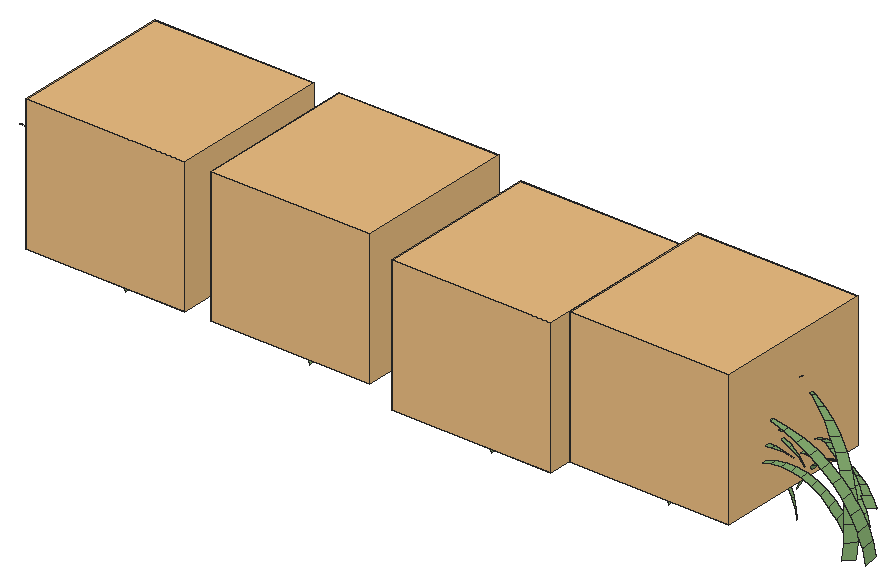
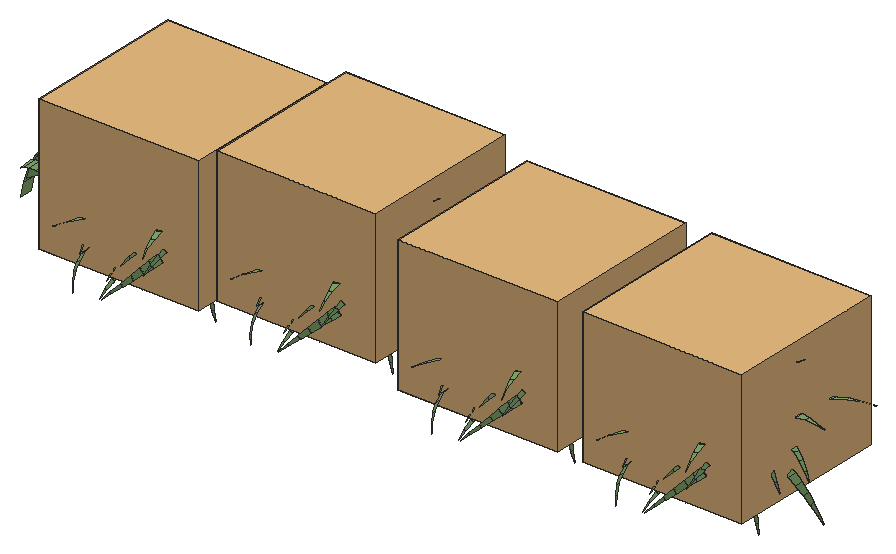
# SketchUp Ruby script. Lengths in inches.
U = 1.inch
M = Sketchup.active_model
def pt(a) = Geom::Point3d.new(a.map { |v| v * U })
def face(e, loops, mat)
  f = e.add_face(loops[0].map { |a| pt(a) })
  loops[1..].each { |l| e.add_face(l.map { |a| pt(a) }).erase! }
  f.material = f.back_material = mat if mat
  f
end
# faces: each face lists its corners as indices into pts; further lists are holes
def faces(e, pts, list, mat = nil) = list.each { |f| face(e, (f[0].is_a?(Array) ? f : [f]).map { |l| l.map { |i| pts[i] } }, mat) }
# xy, xz, yz: faces in a plane at the given z, y or x. An outline is a flat list of corners, or four numbers for a rectangle; further outlines are holes
def ring(l) = l.size == 4 ? [[l[0], l[1]], [l[2], l[1]], [l[2], l[3]], [l[0], l[3]]] : l.each_slice(2).to_a
def flat(e, list, mat, &to3) = list.each { |f| face(e, (f[0].is_a?(Array) ? f : [f]).map { |l| ring(l).map { |u, v| to3.(u, v) } }, mat) }
def xy(e, z, list, mat = nil) = flat(e, list, mat) { |x, y| [x, y, z] }
def xz(e, y, list, mat = nil) = flat(e, list, mat) { |x, z| [x, y, z] }
def yz(e, x, list, mat = nil) = flat(e, list, mat) { |y, z| [x, y, z] }
def lines(e, pts, list) = list.each { |a, b| e.add_line(pt(pts[a]), pt(pts[b])) }
# prism: a flat outline (further loops are holes) pulled along v
def prism(e, loops, v, mat = nil)
  f = face(e, loops, mat); d = Geom::Vector3d.new(v.map { |x| x * U })
  f.pushpull(f.normal.samedirection?(d) ? d.length : -d.length)
end
def box(e, o, s, mat = nil) = prism(e, [[o, [o[0] + s[0], o[1], o[2]], [o[0] + s[0], o[1] + s[1], o[2]], [o[0], o[1] + s[1], o[2]]]], [0, 0, s[2]], mat)
def at(x, y, z, deg = 0) = Geom::Transformation.translation(pt([x, y, z])) * Geom::Transformation.rotation(ORIGIN, Z_AXIS, deg.degrees)
def axes(o, x, y, z) = Geom::Transformation.new([*x, 0, *y, 0, *z, 0, *pt(o).to_a, 1])
def part(name) = M.definitions.add(name)
# library, detail: a bought-in or finely detailed component or shape, given as its bounding box
def library(name, o, s) = part(name).tap { |d| box(d.entities, o, s) }
def detail(e, o, s) = box(e.add_group.entities, o, s)
def put(e, d, t, mat = nil) = e.add_instance(d, t).tap { |i| i.material = mat if mat }
def group(e, t, mat = nil) = e.add_group.tap { |g| g.transformation = t; g.material = mat if mat }.entities
root = M.entities
M.materials.add("dianella").color = [131, 171, 111]
c1 = part("Shape Bender Component\#5")
p = [[0.17,0.01,0.72],[1.09,0.03,4.5625],[1.09,3.73,4.5625],[0.17,3.75,0.72],[2.23,0.05,7.59],[2.48,0.0625,8.26],
  [2.48,3.71,8.26],[2.23,3.72,7.59],[4.33,0.14,11.74],[4.33,3.64,11.74],[6.2,0.2,14.41],[6.6,0.22,14.97],
  [6.6,3.56,14.97],[6.2,3.58,14.41],[9.26,0.35,17.88],[9.26,3.43,17.88],[12.27,0.4,20.43],[12.27,3.38,20.43],
  [15.58,0.51,22.59],[15.58,3.27,22.59],[19.13,0.73,24.3],[19.13,3.14,24.3],[22.875,1.08,25.56],[22.875,2.85,25.56],
  [26.75,1.47,26.33],[26.75,2.49,26.33],[30.68,1.86,26.6],[30.68,2.125,26.6],[33.95,1.875,26.45]]
faces(c1.entities,p,[[0,1,2,3],[1,4,5,6,7,2],[5,8,9,6],[8,10,11,12,13,9],[11,14,15,12],[14,16,17,15],[16,18,19,17],[18,20,21,19],
  [20,22,23,21],[22,24,25,23],[24,26,27,25],[28,27,26]],"dianella")
c2 = part("Shape Bender Component\#4")
p = [[0.27,1.78,0.46],[1.95,1.8,3.35],[1.95,4.67,3.35],[0.27,4.68,0.46],[3.06,1.81,4.8],[3.875,1.84,5.87],
  [3.875,4.64,5.87],[3.06,4.66,4.8],[6,1.9,8],[6,4.58,8],[27.35,3.23,6.09],[25.57,3.4375,7.9],
  [25.57,3.03,7.9],[23.28,2.8,9.61],[23.28,3.67,9.61],[7.08,1.93,8.8],[8.3,1.99,9.69],[8.3,4.5,9.69],
  [7.08,4.55,8.8],[23.04,2.78,9.74],[23.04,3.69,9.74],[20.86,3.86,10.86],[20.86,2.625,10.86],[10.73,2.08,10.92],
  [10.73,4.41,10.92],[12.13,2.13,11.33],[13.24,2.19,11.66],[13.24,4.3,11.66],[12.13,4.36,11.33],[18.35,2.46,11.63],
  [18.35,4.03,11.63],[15.79,2.32,11.89],[17.75,2.42,11.69],[17.75,4.07,11.69],[15.79,4.17,11.89]]
faces(c2.entities,p,[[0,1,2,3],[1,4,5,6,7,2],[5,8,9,6],[10,11,12],[13,12,11,14],[15,16,17,18,9,8],[19,13,14,20,21,22],[16,23,24,17],
  [23,25,26,27,28,24],[29,22,21,30],[31,32,29,30,33,34],[26,31,34,27]],"dianella")
c3 = part("Shape Bender Component\#7")
p = [[0.01,0.94,1.17],[0.04,0.96,6.32],[0.04,4.67,6.32],[0.01,4.68,1.17],[0.42,0.98,10.52],[0.51,1,11.45],
  [0.51,4.64,11.45],[0.42,4.66,10.52],[1.4,1.07,16.52],[1.4,4.57,16.52],[2.48,1.13,20.62],[2.71,1.16,21.49],
  [2.71,4.49,21.49],[2.48,4.52,20.625],[4.4375,1.21,26.32],[4.4375,4.46,26.32],[6.56,1.22,30.98],[6.56,4.47,30.98],
  [9.06,1.29,35.43],[9.06,4.38,35.43],[11.92,1.42,39.64],[11.92,4.23,39.64],[15.13,1.74,43.57],[15.13,4,43.57],
  [18.65,2.08,47.2],[18.65,3.67,47.2],[22.46,2.47,50.5],[22.46,3.14,50.5],[25.84,2.81,52.95]]
faces(c3.entities,p,[[0,1,2,3],[1,4,5,6,7,2],[5,8,9,6],[10,11,12,13,9,8],[11,14,15,12],[14,16,17,15],[16,18,19,17],[18,20,21,19],
  [20,22,23,21],[22,24,25,23],[24,26,27,25],[28,27,26]],"dianella")
c4 = library("Trees & Plants  (59)",[-4.49,-4.79,-0.78],[10.02,10.13,10.22])
put(root,c1,axes([69.61,543.69,296.62],[-0.93269,0.35072,0.09345],[0.32759,0.91741,-0.21384],[0.14796,0.18564,0.96108]))
put(root,c2,axes([69.77,549.83,307.5],[-0.86496,0.14883,-0.43169],[0.33112,0.87778,-0.37014],[-0.36493,0.45373,0.81582]))
put(root,c1,axes([73.72,547.22,295.51],[-0.99701,-0.04566,0.06927],[-0.04139,0.99682,0.07559],[0.05813,-0.05813,0.98368]))
put(root,c2,axes([69.1,547.53,301.82],[-0.88813,0.45112,0.09751],[0.45492,0.89007,0.03168],[0.05813,-0.05813,0.98368]))
put(root,c2,axes([70.16,548.4,303.95],[-0.80569,0.56944,-0.02305],[0.57633,0.79454,-0.18542],[0.07749,0.17806,0.9833]))
put(root,c3,axes([71.76,546.25,295.18],[-0.89818,0.42386,0.09751],[0.36913,0.65726,0.03168],[0.04524,-0.03705,0.72823]))
put(root,c2,axes([67.54,544.48,305.64],[-0.51985,0.69677,-0.46908],[0.85127,0.46792,-0.24029],[-0.06489,0.54284,0.83687]))
put(root,c2,axes([69.68,544.76,295.79],[-0.45461,0.886,-0.06101],[0.85593,0.46132,0.22475],[-0.24461,-0.03601,0.9612]))
put(root,c2,axes([66.4375,554.24,305.89],[-0.07554,0.99436,-0.05049],[0.89319,0.09828,0.42129],[-0.44228,0.02665,0.89336]))
put(root,c1,axes([71.59,550.61,299.04],[-0.33829,0.92096,-0.16447],[0.74479,0.29265,-0.04252],[-0.03806,0.18424,0.97431]))
put(root,c2,axes([67.27,560.98,305.84],[0.17955,0.96457,-0.21457],[0.72432,-0.00444,0.72223],[-0.65717,0.24154,0.6603]))
put(root,c2,axes([71.16,548.68,298.19],[-0.07554,0.99436,-0.05049],[0.89319,0.09828,0.42129],[-0.44228,0.02665,0.89336]))
put(root,c2,axes([68.37,552.72,301.24],[0.15821,0.98591,0.06027],[0.88231,-0.16242,0.42],[-0.44228,0.02665,0.89336]))
put(root,c4,axes([73.47,553.09,306.65],[4.356,0,0],[0,4.356,0],[0,0,3.6]))
put(root,c2,axes([70.07,551.76,296.11],[0.15821,0.98591,0.06027],[0.98524,-0.15399,-0.08295],[0.05813,-0.05813,0.98368]))
put(root,c2,axes([72.25,546.79,295.83],[0.26556,0.96121,-0.04549],[-0.85756,0.2684,0.37954],[0.43914,-0.059,0.80483]))
put(root,c2,axes([75.77,550.21,298.58],[0.03456,0.99793,0.05429],[-0.89708,0.01048,0.37838],[0.43914,-0.059,0.80483]))
put(root,c2,axes([80.06,553.69,293.96],[0.03456,0.99793,0.05429],[-0.99646,0.03857,-0.07473],[-0.06824,-0.04585,0.88619]))
put(root,c1,axes([71.4,548.07,296.59],[0.52067,0.83248,-0.14817],[-0.85026,0.52497,-0.03831],[0.06887,0.17559,0.87775]))
put(root,c2,axes([72.94,542.66,293.66],[0.61668,0.7819,-0.05497],[-0.7511,0.61748,0.20248],[0.2331,-0.08243,0.86594]))
put(root,c2,axes([78.43,558.11,302.72],[0.00951,0.98109,-0.1933],[-0.71163,0.13509,0.65066],[0.69138,0.1105,0.59486]))
put(root,c2,axes([77.95,551.34,302.77],[0.26556,0.96121,-0.04549],[-0.85756,0.2684,0.37954],[0.43914,-0.059,0.80483]))
put(root,c2,axes([72.34,546.12,299.32],[0.87579,0.38306,0.08831],[-0.40412,0.89443,-0.16738],[-0.06046,0.18068,0.91811]))
put(root,c3,axes([73.24,557.07,294.86],[0.94689,0.23499,0.20991],[0.15697,-0.72589,-0.13304],[-0.09792,-0.17134,0.70342]))
put(root,c2,axes([74.95,549.02,305.54],[0.82667,0.29857,0.38049],[-0.23842,0.92604,-0.27787],[-0.34507,0.20027,0.85088]))
put(root,c3,axes([73.66,553.52,294.52],[0.80902,-0.58527,0.05755],[-0.58572,-0.79585,0.15754],[0.03689,0.112,0.69708]))
put(root,c3,axes([77.36,548.43,293.12],[0.95837,0.27169,0.08785],[-0.27506,0.961,0.02854],[-0.05052,-0.03395,0.65606]))
put(root,c1,axes([71.12,552.34,294.5],[0.99357,-0.11272,0.01108],[-0.1132,-0.98932,0.09728],[0,0.08221,0.93937]))
put(root,c2,axes([73.84,547.65,304.22],[0.87743,-0.02048,-0.38891],[-0.15593,0.92511,-0.33346],[0.44545,0.37499,0.73497]))
put(root,c2,axes([76.85,552.81,306.52],[1,0,0],[0,-0.99572,0.09791],[0,0.08221,0.93937]))
put(root,c1,axes([75.6,549.94,293.42],[0.96956,-0.23675,0.0624],[0.23253,0.9702,0.0681],[-0.06824,-0.04585,0.88619]))
put(root,c2,axes([80.1875,549.36,299.1],[0.95837,0.27169,0.08785],[-0.27506,0.961,0.02854],[-0.06824,-0.04585,0.88619]))
put(root,c1,axes([120.13,543.69,296.62],[-0.93269,0.35072,0.09345],[0.32759,0.91741,-0.21384],[0.14796,0.18564,0.96108]))
put(root,c2,axes([120.29,549.83,307.5],[-0.86496,0.14883,-0.43169],[0.33112,0.87778,-0.37014],[-0.36493,0.45373,0.81582]))
put(root,c2,axes([119.62,547.53,301.82],[-0.88813,0.45112,0.09751],[0.45492,0.89007,0.03168],[0.05813,-0.05813,0.98368]))
put(root,c2,axes([120.68,548.4,303.95],[-0.80569,0.56944,-0.02305],[0.57633,0.79454,-0.18542],[0.07749,0.17806,0.9833]))
put(root,c2,axes([118.06,544.48,305.64],[-0.51985,0.69677,-0.46908],[0.85127,0.46792,-0.24029],[-0.06489,0.54284,0.83687]))
put(root,c2,axes([120.2,544.76,295.79],[-0.45461,0.886,-0.06101],[0.85593,0.46132,0.22475],[-0.24461,-0.03601,0.9612]))
put(root,c2,axes([116.96,554.24,305.89],[-0.07554,0.99436,-0.05049],[0.89319,0.09828,0.42129],[-0.44228,0.02665,0.89336]))
put(root,c1,axes([122.11,550.61,299.04],[-0.33829,0.92096,-0.16447],[0.74479,0.29265,-0.04252],[-0.03806,0.18424,0.97431]))
put(root,c2,axes([117.79,560.98,305.84],[0.17955,0.96457,-0.21457],[0.72432,-0.00444,0.72223],[-0.65717,0.24154,0.6603]))
put(root,c2,axes([118.89,552.72,301.24],[0.15821,0.98591,0.06027],[0.88231,-0.16242,0.42],[-0.44228,0.02665,0.89336]))
put(root,c4,axes([123.99,553.09,306.65],[4.356,0,0],[0,4.356,0],[0,0,3.6]))
put(root,c2,axes([120.59,551.76,296.11],[0.15821,0.98591,0.06027],[0.98524,-0.15399,-0.08295],[0.05813,-0.05813,0.98368]))
put(root,c2,axes([122.77,546.79,295.83],[0.26556,0.96121,-0.04549],[-0.85756,0.2684,0.37954],[0.43914,-0.059,0.80483]))
put(root,c2,axes([126.29,550.21,298.58],[0.03456,0.99793,0.05429],[-0.89708,0.01048,0.37838],[0.43914,-0.059,0.80483]))
put(root,c2,axes([130.58,553.69,293.96],[0.03456,0.99793,0.05429],[-0.99646,0.03857,-0.07473],[-0.06824,-0.04585,0.88619]))
put(root,c1,axes([121.92,548.07,296.59],[0.52067,0.83248,-0.14817],[-0.85026,0.52497,-0.03831],[0.06887,0.17559,0.87775]))
put(root,c2,axes([123.46,542.66,293.66],[0.61668,0.7819,-0.05497],[-0.7511,0.61748,0.20248],[0.2331,-0.08243,0.86594]))
put(root,c2,axes([128.95,558.11,302.72],[0.00951,0.98109,-0.1933],[-0.71163,0.13509,0.65066],[0.69138,0.1105,0.59486]))
put(root,c2,axes([128.47,551.34,302.77],[0.26556,0.96121,-0.04549],[-0.85756,0.2684,0.37954],[0.43914,-0.059,0.80483]))
put(root,c2,axes([122.86,546.12,299.32],[0.87579,0.38306,0.08831],[-0.40412,0.89443,-0.16738],[-0.06046,0.18068,0.91811]))
put(root,c3,axes([123.76,557.07,294.86],[0.94689,0.23499,0.20991],[0.15697,-0.72589,-0.13304],[-0.09792,-0.17134,0.70342]))
put(root,c2,axes([125.47,549.02,305.54],[0.82667,0.29857,0.38049],[-0.23842,0.92604,-0.27787],[-0.34507,0.20027,0.85088]))
put(root,c3,axes([124.18,553.52,294.52],[0.80902,-0.58527,0.05755],[-0.58572,-0.79585,0.15754],[0.03689,0.112,0.69708]))
put(root,c3,axes([127.88,548.43,293.12],[0.95837,0.27169,0.08785],[-0.27506,0.961,0.02854],[-0.05052,-0.03395,0.65606]))
put(root,c1,axes([121.64,552.34,294.5],[0.99357,-0.11272,0.01108],[-0.1132,-0.98932,0.09728],[0,0.08221,0.93937]))
put(root,c2,axes([124.36,547.65,304.22],[0.87743,-0.02048,-0.38891],[-0.15593,0.92511,-0.33346],[0.44545,0.37499,0.73497]))
put(root,c2,axes([127.37,552.81,306.52],[1,0,0],[0,-0.99572,0.09791],[0,0.08221,0.93937]))
put(root,c1,axes([126.12,549.94,293.42],[0.96956,-0.23675,0.0624],[0.23253,0.9702,0.0681],[-0.06824,-0.04585,0.88619]))
put(root,c2,axes([130.71,549.36,299.1],[0.95837,0.27169,0.08785],[-0.27506,0.961,0.02854],[-0.06824,-0.04585,0.88619]))
put(root,c1,axes([174.61,537.69,296.62],[-0.93269,0.35072,0.09345],[0.32759,0.91741,-0.21384],[0.14796,0.18564,0.96108]))
put(root,c2,axes([174.77,543.83,307.5],[-0.86496,0.14883,-0.43169],[0.33112,0.87778,-0.37014],[-0.36493,0.45373,0.81582]))
put(root,c2,axes([174.11,541.53,301.82],[-0.88813,0.45112,0.09751],[0.45492,0.89007,0.03168],[0.05813,-0.05813,0.98368]))
put(root,c2,axes([175.17,542.4,303.95],[-0.80569,0.56944,-0.02305],[0.57633,0.79454,-0.18542],[0.07749,0.17806,0.9833]))
put(root,c3,axes([176.76,540.25,295.18],[-0.89818,0.42386,0.09751],[0.36913,0.65726,0.03168],[0.04524,-0.03705,0.72823]))
put(root,c2,axes([172.54,538.48,305.64],[-0.51985,0.69677,-0.46908],[0.85127,0.46792,-0.24029],[-0.06489,0.54284,0.83687]))
put(root,c2,axes([174.6875,538.76,295.79],[-0.45461,0.886,-0.06101],[0.85593,0.46132,0.22475],[-0.24461,-0.03601,0.9612]))
put(root,c2,axes([171.44,548.24,305.89],[-0.07554,0.99436,-0.05049],[0.89319,0.09828,0.42129],[-0.44228,0.02665,0.89336]))
put(root,c1,axes([176.6,544.61,299.04],[-0.33829,0.92096,-0.16447],[0.74479,0.29265,-0.04252],[-0.03806,0.18424,0.97431]))
put(root,c2,axes([172.28,554.98,305.84],[0.17955,0.96457,-0.21457],[0.72432,-0.00444,0.72223],[-0.65717,0.24154,0.6603]))
put(root,c2,axes([176.16,542.68,298.19],[-0.07554,0.99436,-0.05049],[0.89319,0.09828,0.42129],[-0.44228,0.02665,0.89336]))
put(root,c2,axes([173.37,546.72,301.24],[0.15821,0.98591,0.06027],[0.88231,-0.16242,0.42],[-0.44228,0.02665,0.89336]))
put(root,c4,axes([178.47,547.09,306.65],[4.356,0,0],[0,4.356,0],[0,0,3.6]))
put(root,c2,axes([175.07,545.76,296.11],[0.15821,0.98591,0.06027],[0.98524,-0.15399,-0.08295],[0.05813,-0.05813,0.98368]))
put(root,c2,axes([177.25,540.79,295.83],[0.26556,0.96121,-0.04549],[-0.85756,0.2684,0.37954],[0.43914,-0.059,0.80483]))
put(root,c2,axes([180.77,544.21,298.58],[0.03456,0.99793,0.05429],[-0.89708,0.01048,0.37838],[0.43914,-0.059,0.80483]))
put(root,c2,axes([185.06,547.69,293.96],[0.03456,0.99793,0.05429],[-0.99646,0.03857,-0.07473],[-0.06824,-0.04585,0.88619]))
put(root,c1,axes([176.41,542.07,296.59],[0.52067,0.83248,-0.14817],[-0.85026,0.52497,-0.03831],[0.06887,0.17559,0.87775]))
put(root,c2,axes([177.95,536.66,293.66],[0.61668,0.7819,-0.05497],[-0.7511,0.61748,0.20248],[0.2331,-0.08243,0.86594]))
put(root,c2,axes([183.4375,552.11,302.72],[0.00951,0.98109,-0.1933],[-0.71163,0.13509,0.65066],[0.69138,0.1105,0.59486]))
put(root,c2,axes([182.95,545.34,302.77],[0.26556,0.96121,-0.04549],[-0.85756,0.2684,0.37954],[0.43914,-0.059,0.80483]))
put(root,c2,axes([177.35,540.12,299.32],[0.87579,0.38306,0.08831],[-0.40412,0.89443,-0.16738],[-0.06046,0.18068,0.91811]))
put(root,c3,axes([178.25,551.07,294.86],[0.94689,0.23499,0.20991],[0.15697,-0.72589,-0.13304],[-0.09792,-0.17134,0.70342]))
put(root,c2,axes([179.95,543.02,305.54],[0.82667,0.29857,0.38049],[-0.23842,0.92604,-0.27787],[-0.34507,0.20027,0.85088]))
put(root,c3,axes([182.37,542.43,293.12],[0.95837,0.27169,0.08785],[-0.27506,0.961,0.02854],[-0.05052,-0.03395,0.65606]))
put(root,c2,axes([178.84,541.65,304.22],[0.87743,-0.02048,-0.38891],[-0.15593,0.92511,-0.33346],[0.44545,0.37499,0.73497]))
put(root,c2,axes([185.19,543.36,299.1],[0.95837,0.27169,0.08785],[-0.27506,0.961,0.02854],[-0.06824,-0.04585,0.88619]))
put(root,c1,axes([218.53,543.69,296.62],[-0.93269,0.35072,0.09345],[0.32759,0.91741,-0.21384],[0.14796,0.18564,0.96108]))
put(root,c2,axes([218.69,549.83,307.5],[-0.86496,0.14883,-0.43169],[0.33112,0.87778,-0.37014],[-0.36493,0.45373,0.81582]))
put(root,c1,axes([222.64,547.22,295.51],[-0.99701,-0.04566,0.06927],[-0.04139,0.99682,0.07559],[0.05813,-0.05813,0.98368]))
put(root,c2,axes([218.03,547.53,301.82],[-0.88813,0.45112,0.09751],[0.45492,0.89007,0.03168],[0.05813,-0.05813,0.98368]))
put(root,c2,axes([219.09,548.4,303.95],[-0.80569,0.56944,-0.02305],[0.57633,0.79454,-0.18542],[0.07749,0.17806,0.9833]))
put(root,c3,axes([220.68,546.25,295.18],[-0.89818,0.42386,0.09751],[0.36913,0.65726,0.03168],[0.04524,-0.03705,0.72823]))
put(root,c2,axes([216.46,544.48,305.64],[-0.51985,0.69677,-0.46908],[0.85127,0.46792,-0.24029],[-0.06489,0.54284,0.83687]))
put(root,c2,axes([218.61,544.76,295.79],[-0.45461,0.886,-0.06101],[0.85593,0.46132,0.22475],[-0.24461,-0.03601,0.9612]))
put(root,c2,axes([215.36,554.24,305.89],[-0.07554,0.99436,-0.05049],[0.89319,0.09828,0.42129],[-0.44228,0.02665,0.89336]))
put(root,c1,axes([220.52,550.61,299.04],[-0.33829,0.92096,-0.16447],[0.74479,0.29265,-0.04252],[-0.03806,0.18424,0.97431]))
put(root,c2,axes([216.2,560.98,305.84],[0.17955,0.96457,-0.21457],[0.72432,-0.00444,0.72223],[-0.65717,0.24154,0.6603]))
put(root,c2,axes([220.08,548.68,298.19],[-0.07554,0.99436,-0.05049],[0.89319,0.09828,0.42129],[-0.44228,0.02665,0.89336]))
put(root,c2,axes([217.29,552.72,301.24],[0.15821,0.98591,0.06027],[0.88231,-0.16242,0.42],[-0.44228,0.02665,0.89336]))
put(root,c4,axes([222.39,553.09,306.65],[4.356,0,0],[0,4.356,0],[0,0,3.6]))
put(root,c2,axes([218.99,551.76,296.11],[0.15821,0.98591,0.06027],[0.98524,-0.15399,-0.08295],[0.05813,-0.05813,0.98368]))
put(root,c2,axes([221.17,546.79,295.83],[0.26556,0.96121,-0.04549],[-0.85756,0.2684,0.37954],[0.43914,-0.059,0.80483]))
put(root,c2,axes([224.69,550.21,298.58],[0.03456,0.99793,0.05429],[-0.89708,0.01048,0.37838],[0.43914,-0.059,0.80483]))
put(root,c2,axes([228.98,553.69,293.96],[0.03456,0.99793,0.05429],[-0.99646,0.03857,-0.07473],[-0.06824,-0.04585,0.88619]))
put(root,c1,axes([220.33,548.07,296.59],[0.52067,0.83248,-0.14817],[-0.85026,0.52497,-0.03831],[0.06887,0.17559,0.87775]))
put(root,c2,axes([221.87,542.66,293.66],[0.61668,0.7819,-0.05497],[-0.7511,0.61748,0.20248],[0.2331,-0.08243,0.86594]))
put(root,c2,axes([227.36,558.11,302.72],[0.00951,0.98109,-0.1933],[-0.71163,0.13509,0.65066],[0.69138,0.1105,0.59486]))
put(root,c2,axes([226.875,551.34,302.77],[0.26556,0.96121,-0.04549],[-0.85756,0.2684,0.37954],[0.43914,-0.059,0.80483]))
put(root,c2,axes([221.27,546.12,299.32],[0.87579,0.38306,0.08831],[-0.40412,0.89443,-0.16738],[-0.06046,0.18068,0.91811]))
put(root,c3,axes([222.17,557.07,294.86],[0.94689,0.23499,0.20991],[0.15697,-0.72589,-0.13304],[-0.09792,-0.17134,0.70342]))
put(root,c2,axes([223.875,549.02,305.54],[0.82667,0.29857,0.38049],[-0.23842,0.92604,-0.27787],[-0.34507,0.20027,0.85088]))
put(root,c3,axes([222.58,553.52,294.52],[0.80902,-0.58527,0.05755],[-0.58572,-0.79585,0.15754],[0.03689,0.112,0.69708]))
put(root,c3,axes([226.29,548.43,293.12],[0.95837,0.27169,0.08785],[-0.27506,0.961,0.02854],[-0.05052,-0.03395,0.65606]))
put(root,c1,axes([220.05,552.34,294.5],[0.99357,-0.11272,0.01108],[-0.1132,-0.98932,0.09728],[0,0.08221,0.93937]))
put(root,c2,axes([222.76,547.65,304.22],[0.87743,-0.02048,-0.38891],[-0.15593,0.92511,-0.33346],[0.44545,0.37499,0.73497]))
put(root,c2,axes([225.77,552.81,306.52],[1,0,0],[0,-0.99572,0.09791],[0,0.08221,0.93937]))
put(root,c1,axes([224.52,549.94,293.42],[0.96956,-0.23675,0.0624],[0.23253,0.9702,0.0681],[-0.06824,-0.04585,0.88619]))
put(root,c2,axes([229.11,549.36,299.1],[0.95837,0.27169,0.08785],[-0.27506,0.961,0.02854],[-0.06824,-0.04585,0.88619]))
put(root,c2,axes([267.07,544.77,301.91],[-0.98591,-0.15821,0.06027],[-0.15399,0.98524,0.08295],[0.05813,-0.05813,0.98368]))
put(root,c1,axes([268.09,543.69,296.62],[-0.93269,0.35072,0.09345],[0.32759,0.91741,-0.21384],[0.14796,0.18564,0.96108]))
put(root,c2,axes([268.25,549.83,307.5],[-0.86496,0.14883,-0.43169],[0.33112,0.87778,-0.37014],[-0.36493,0.45373,0.81582]))
put(root,c1,axes([272.2,547.22,295.51],[-0.99701,-0.04566,0.06927],[-0.04139,0.99682,0.07559],[0.05813,-0.05813,0.98368]))
put(root,c2,axes([267.59,547.53,301.82],[-0.88813,0.45112,0.09751],[0.45492,0.89007,0.03168],[0.05813,-0.05813,0.98368]))
